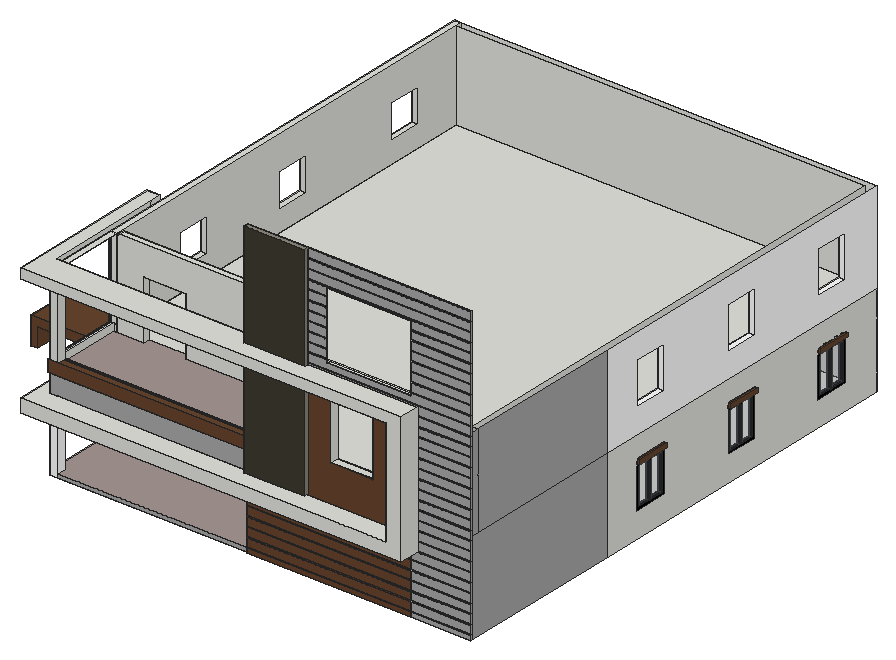
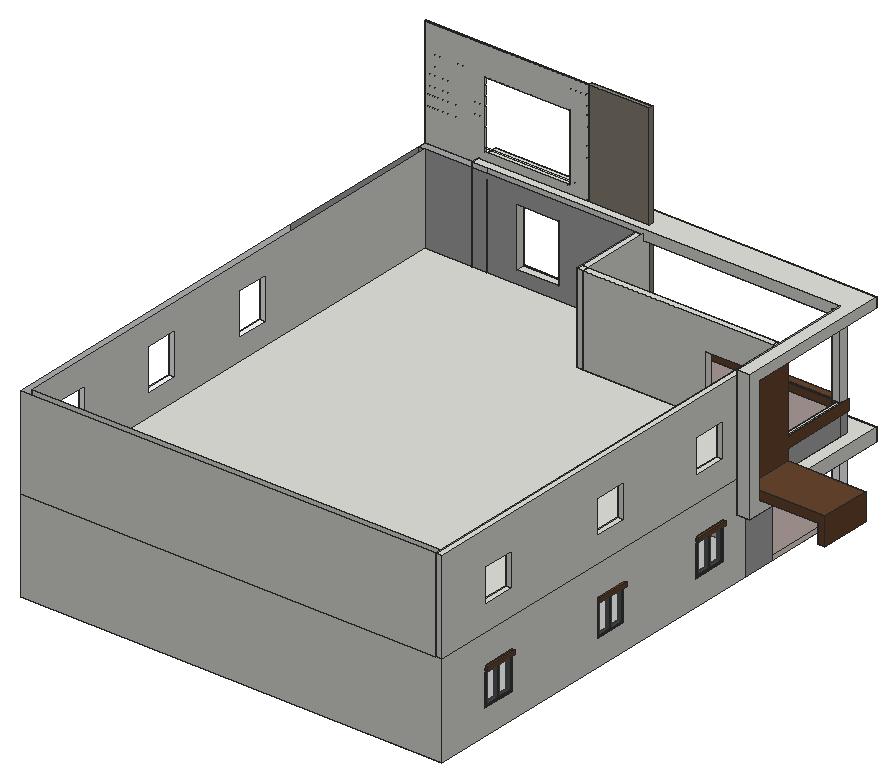
# SketchUp Ruby script. Lengths in inches.
U = 1.inch
M = Sketchup.active_model
def pt(a) = Geom::Point3d.new(a.map { |v| v * U })
def face(e, loops, mat)
  f = e.add_face(loops[0].map { |a| pt(a) })
  loops[1..].each { |l| e.add_face(l.map { |a| pt(a) }).erase! }
  f.material = f.back_material = mat if mat
  f
end
# faces: each face lists its corners as indices into pts; further lists are holes
def faces(e, pts, list, mat = nil) = list.each { |f| face(e, (f[0].is_a?(Array) ? f : [f]).map { |l| l.map { |i| pts[i] } }, mat) }
# xy, xz, yz: faces in a plane at the given z, y or x. An outline is a flat list of corners, or four numbers for a rectangle; further outlines are holes
def ring(l) = l.size == 4 ? [[l[0], l[1]], [l[2], l[1]], [l[2], l[3]], [l[0], l[3]]] : l.each_slice(2).to_a
def flat(e, list, mat, &to3) = list.each { |f| face(e, (f[0].is_a?(Array) ? f : [f]).map { |l| ring(l).map { |u, v| to3.(u, v) } }, mat) }
def xy(e, z, list, mat = nil) = flat(e, list, mat) { |x, y| [x, y, z] }
def xz(e, y, list, mat = nil) = flat(e, list, mat) { |x, z| [x, y, z] }
def yz(e, x, list, mat = nil) = flat(e, list, mat) { |y, z| [x, y, z] }
def lines(e, pts, list) = list.each { |a, b| e.add_line(pt(pts[a]), pt(pts[b])) }
# prism: a flat outline (further loops are holes) pulled along v
def prism(e, loops, v, mat = nil)
  f = face(e, loops, mat); d = Geom::Vector3d.new(v.map { |x| x * U })
  f.pushpull(f.normal.samedirection?(d) ? d.length : -d.length)
end
def box(e, o, s, mat = nil) = prism(e, [[o, [o[0] + s[0], o[1], o[2]], [o[0] + s[0], o[1] + s[1], o[2]], [o[0], o[1] + s[1], o[2]]]], [0, 0, s[2]], mat)
def at(x, y, z, deg = 0) = Geom::Transformation.translation(pt([x, y, z])) * Geom::Transformation.rotation(ORIGIN, Z_AXIS, deg.degrees)
def axes(o, x, y, z) = Geom::Transformation.new([*x, 0, *y, 0, *z, 0, *pt(o).to_a, 1])
def part(name) = M.definitions.add(name)
# library, detail: a bought-in or finely detailed component or shape, given as its bounding box
def library(name, o, s) = part(name).tap { |d| box(d.entities, o, s) }
def detail(e, o, s) = box(e.add_group.entities, o, s)
def put(e, d, t, mat = nil) = e.add_instance(d, t).tap { |i| i.material = mat if mat }
def group(e, t, mat = nil) = e.add_group.tap { |g| g.transformation = t; g.material = mat if mat }.entities
root = M.entities
M.materials.add("Glass_Basic_01").color = [161, 173, 186]
M.materials["Glass_Basic_01"].alpha = 0.25
M.materials.add("M00_Soft_Cloud").color = [255, 255, 255]
M.materials.add("M03_Pewter_Shine").color = [168, 168, 168]
M.materials.add("M07_Charcoal_Gleam").color = [58, 58, 58]
M.materials.add("M09_Shadow_Night").color = [0, 0, 0]
M.materials.add("Marble_01_1K").color = [230, 221, 211]
M.materials.add("Marble_06_1K").color = [165, 150, 147]
M.materials.add("Metal_06_1K").color = [238, 236, 231]
M.materials.add("Plaster_06_1K").color = [141, 135, 122]
M.materials.add("Tile_Exterior_07_1K").color = [112, 111, 107]
M.materials.add("Tile_Exterior_08_1K").color = [62, 60, 47]
M.materials.add("Wood_Veneer_15_1K").color = [103, 69, 45]
c1 = library("Group\#33",[0,0,0],[60,6,84])
c2 = part("Stair tread")
xy(c2.entities,3,[[0,0,10,60]],"Wood_Veneer_15_1K")
xy(c2.entities,6,[[0,0,10,60]],"Wood_Veneer_15_1K")
xz(c2.entities,0,[[0,3,10,6]],"Wood_Veneer_15_1K")
xz(c2.entities,60,[[0,3,10,6]])
yz(c2.entities,0,[[0,3,60,6]],"Wood_Veneer_15_1K")
yz(c2.entities,10,[[0,3,60,6]],"Wood_Veneer_15_1K")
c3 = part("Tread with baluster")
box(c3.entities,[0,0,3],[10,60,3])
g1 = group(c3.entities,at(3.7,1.6875,6))
prism(g1,[[[0.9375,0,0],[0.69,0.03,0],[0.47,0.125,0],[0.27,0.27,0],[0.125,0.47,0],[0.03,0.69,0],[0,0.9375,0],[0.03,1.18,0],[0.125,1.41,0],[0.27,1.6,0],[0.47,1.75,0],[0.69,1.84,0],[0.9375,1.875,0],[1.18,1.84,0],[1.41,1.75,0],[1.6,1.6,0],[1.75,1.41,0],[1.84,1.18,0],[1.875,0.9375,0],[1.84,0.69,0],[1.75,0.47,0],[1.6,0.27,0],[1.41,0.125,0],[1.18,0.03,0]]],[0,0,36.125],"Metal_06_1K")
c4 = part("Group\#49")
put(c4.entities,c2,at(70,0,87))
put(c4.entities,c2,at(60,0,93))
put(c4.entities,c2,at(30,0,111))
put(c4.entities,c2,at(90,0,75))
put(c4.entities,c2,at(10,0,123))
put(c4.entities,c2,at(20,0,117))
put(c4.entities,c2,at(50,0,99))
put(c4.entities,c2,at(40,0,105))
put(c4.entities,c2,at(100,0,69))
put(c4.entities,c2,at(80,0,81))
put(c4.entities,c3,at(100,60,57),"Wood_Veneer_15_1K")
put(c4.entities,c3,at(40,60,21),"Wood_Veneer_15_1K")
put(c4.entities,c3,at(60,60,33),"Wood_Veneer_15_1K")
put(c4.entities,c3,at(80,60,45),"Wood_Veneer_15_1K")
put(c4.entities,c3,at(90,60,51),"Wood_Veneer_15_1K")
put(c4.entities,c3,at(70,60,39),"Wood_Veneer_15_1K")
put(c4.entities,c3,at(10,60,3),"Wood_Veneer_15_1K")
put(c4.entities,c3,at(50,60,27),"Wood_Veneer_15_1K")
put(c4.entities,c3,at(30,60,15),"Wood_Veneer_15_1K")
put(c4.entities,c3,at(0,60,-3),"Wood_Veneer_15_1K")
put(c4.entities,c3,at(20,60,9),"Wood_Veneer_15_1K")
g2 = group(c4.entities,at(110,60,63),"Wood_Veneer_15_1K")
box(g2,[0,-60,0],[70,120,6])
c5 = part("Group\#23")
xy(c5.entities,0,[[-6,0,0,48]],"M07_Charcoal_Gleam")
xy(c5.entities,3,[[-6,3,0,23],[-6,25,0,45]],"M07_Charcoal_Gleam")
xy(c5.entities,45,[[-6,3,0,23],[-6,25,0,45]],"M07_Charcoal_Gleam")
xy(c5.entities,48,[[-6,0,0,48]],"M07_Charcoal_Gleam")
xz(c5.entities,0,[[-6,0,0,48]],"M07_Charcoal_Gleam")
xz(c5.entities,3,[[-6,3,0,45]],"M07_Charcoal_Gleam")
xz(c5.entities,23,[[-6,3,0,45]],"M07_Charcoal_Gleam")
xz(c5.entities,25,[[-6,3,0,45]],"M07_Charcoal_Gleam")
xz(c5.entities,45,[[-6,3,0,45]],"M07_Charcoal_Gleam")
xz(c5.entities,48,[[-6,0,0,48]],"M07_Charcoal_Gleam")
yz(c5.entities,-6,[[3,3,23,45],[25,3,45,45]],"Glass_Basic_01")
yz(c5.entities,-6,[[[0,0,48,48],[3,3,45,45]],[23,3,25,45]],"M07_Charcoal_Gleam")
yz(c5.entities,0,[[[0,0,48,48],[25,3,45,45],[3,3,23,45]]],"M07_Charcoal_Gleam")
c6 = part("Group\#21")
xy(c6.entities,0,[[0,0,6,48]],"M09_Shadow_Night")
xy(c6.entities,3,[[0,3,6,23],[0,25,6,45]],"M09_Shadow_Night")
xy(c6.entities,56.625,[[0,3,6,23],[0,25,6,45]],"M09_Shadow_Night")
xy(c6.entities,59.625,[[0,0,6,48]],"M09_Shadow_Night")
xz(c6.entities,0,[[0,0,6,59.625]],"M09_Shadow_Night")
xz(c6.entities,3,[[0,3,6,56.625]],"M09_Shadow_Night")
xz(c6.entities,23,[[0,3,6,56.625]],"M09_Shadow_Night")
xz(c6.entities,25,[[0,3,6,56.625]],"M09_Shadow_Night")
xz(c6.entities,45,[[0,3,6,56.625]],"M09_Shadow_Night")
xz(c6.entities,48,[[0,0,6,59.625]],"M09_Shadow_Night")
yz(c6.entities,0,[[[0,0,48,59.625],[25,3,45,56.625],[3,3,23,56.625]]],"M09_Shadow_Night")
yz(c6.entities,6,[[3,3,23,56.625],[25,3,45,56.625]],"Glass_Basic_01")
yz(c6.entities,6,[[[0,0,48,59.625],[3,3,45,56.625]],[23,3,25,56.625]],"M09_Shadow_Night")
c7 = part("Group\#22")
box(c7.entities,[-4,0,0],[4,48,6],"Wood_Veneer_15_1K")
g3 = group(root,at(8950.9375,4405.5625,18))
xy(g3,0,[[0,0,600,720]])
xy(g3,6,[[287.43,12,591,12,591,711,9,711,9,140.1,287.43,140.1]])
xy(g3,6,[[12,0,281.43,0,281.43,134.1,110.3125,134.1,110.3125,140.1,50.3125,140.1,50.3125,134.1,0,134.1,0,12,12,12]],"Marble_06_1K")
xy(g3,36,[[0,220.125,9,268.125],[591,294.5625,600,342.5625],[0,396.5,9,444.5],[591,456.0625,600,504.0625],[0,595.3125,9,643.3125],
  [591,616.5625,600,664.5625]])
xy(g3,84,[[0,220.125,9,268.125],[0,396.5,9,444.5],[0,595.3125,9,643.3125]])
xy(g3,90,[[50.3125,134.1,110.3125,140.1]])
xy(g3,96,[[591,294.5625,600,342.5625],[591,456.0625,600,504.0625],[591,616.5625,600,664.5625]])
xy(g3,104.53,[[12,0,281.43,12],[0,12,9,134.1],[9,12,281.43,134.1]])
xy(g3,131.625,[[0,0,12,0,12,6.5625,9,6.5625,9,12,0,12],[9,6.5625,12,12],[281.43,12,287.43,134.1],[9,134.1,287.43,140.1]])
xy(g3,132,[[12,0,600,0,600,720,0,720,0,12,9,12,9,711,591,711,591,12,12,12],[9,6.5625,12,12]])
xz(g3,0,[[0,0,12,95.53]],"M00_Soft_Cloud")
xz(g3,0,[[12,0,600,0,600,132,12,132,12,131.625,0,131.625,0,95.53,12,95.53,12,104.53,281.43,104.53,281.43,6,12,6]],"M03_Pewter_Shine")
xz(g3,6.5625,[[9,131.625,12,132]])
xz(g3,12,[[287.43,6,287.43,131.625,281.43,131.625,281.43,104.53,9,104.53,9,131.625,12,131.625,12,132,591,132,591,6],[0,131.625,9,132],[9,131.625,12,132]])
xz(g3,12,[[0,6,12,104.53]],"M00_Soft_Cloud")
xz(g3,134.1,[[0,6,50.3125,6,50.3125,90,110.3125,90,110.3125,6,281.43,6,281.43,104.53,0,104.53],[281.43,6,287.43,104.53],[9,104.53,281.43,131.625],[281.43,104.53,287.43,131.625]])
xz(g3,140.1,[[9,6,9,131.625,287.43,131.625,287.43,6,110.3125,6,110.3125,90,50.3125,90,50.3125,6]])
xz(g3,220.125,[[0,36,9,84]])
xz(g3,268.125,[[0,36,9,84]])
xz(g3,294.5625,[[591,36,600,96]])
xz(g3,342.5625,[[591,36,600,96]])
xz(g3,396.5,[[0,36,9,84]])
xz(g3,444.5,[[0,36,9,84]])
xz(g3,456.0625,[[591,36,600,96]])
xz(g3,504.0625,[[591,36,600,96]])
xz(g3,595.3125,[[0,36,9,84]])
xz(g3,616.5625,[[591,36,600,96]])
xz(g3,643.3125,[[0,36,9,84]])
xz(g3,664.5625,[[591,36,600,96]])
xz(g3,711,[[9,6,591,132]])
xz(g3,720,[[0,0,600,132]])
yz(g3,0,[[[179.8125,0,720,132],[220.125,36,268.125,84],[396.5,36,444.5,84],[595.3125,36,643.3125,84]]])
yz(g3,0,[[0,0,12,95.53]],"M00_Soft_Cloud")
yz(g3,0,[[134.1,0,134.1,104.53,12,104.53,12,132,179.8125,132,179.8125,0],[0,95.53,12,131.625]],"M03_Pewter_Shine")
yz(g3,0,[[12,0,134.1,6]],"Marble_01_1K")
yz(g3,9,[[[140.1,6,711,6,711,132,12,132,12,104.53,134.1,104.53,134.1,131.625,140.1,131.625],[220.125,36,268.125,84],[396.5,36,444.5,84],[595.3125,36,643.3125,84]],[6.5625,131.625,12,132]])
yz(g3,12,[[0,131.625,6.5625,132],[6.5625,131.625,12,132]])
yz(g3,12,[[0,6,12,104.53]],"M00_Soft_Cloud")
yz(g3,50.3125,[[134.1,6,140.1,90]])
yz(g3,110.3125,[[134.1,6,140.1,90]])
yz(g3,281.43,[[0,6,134.1,104.53],[12,104.53,134.1,131.625]])
yz(g3,287.43,[[12,6,134.1,131.625],[134.1,6,140.1,131.625]])
yz(g3,591,[[[12,6,711,132],[294.5625,36,342.5625,96],[456.0625,36,504.0625,96],[616.5625,36,664.5625,96]]])
yz(g3,600,[[[240,0,720,132],[294.5625,36,342.5625,96],[456.0625,36,504.0625,96],[616.5625,36,664.5625,96]]])
yz(g3,600,[[0,0,240,132]],"M03_Pewter_Shine")
g4 = group(root,at(9465.6,4405.5625,18))
xy(g4,0,[[0,-0.91,85.34,0]],"M03_Pewter_Shine")
xy(g4,6.0625,[[0,-0.91,85.34,-0.29]],"M09_Shadow_Night")
xy(g4,8.0625,[[0,-0.91,85.34,-0.29]],"M09_Shadow_Night")
xy(g4,19.37,[[0,-0.91,85.34,-0.29]],"M09_Shadow_Night")
xy(g4,21.37,[[0,-0.91,85.34,-0.29]],"M09_Shadow_Night")
xy(g4,32.68,[[0,-0.91,85.34,-0.29]],"M09_Shadow_Night")
xy(g4,34.68,[[0,-0.91,85.34,-0.29]],"M09_Shadow_Night")
xy(g4,45.98,[[0,-0.91,85.34,-0.29]],"M09_Shadow_Night")
xy(g4,47.98,[[0,-0.91,85.34,-0.29]],"M09_Shadow_Night")
xy(g4,59.29,[[0,-0.91,85.34,-0.29]],"M09_Shadow_Night")
xy(g4,61.29,[[0,-0.91,85.34,-0.29]],"M09_Shadow_Night")
xy(g4,72.59,[[0,-0.91,85.34,-0.29]],"M09_Shadow_Night")
xy(g4,74.59,[[0,-0.91,85.34,-0.29]],"M09_Shadow_Night")
xy(g4,85.9,[[0,-0.91,85.34,-0.29]],"M09_Shadow_Night")
xy(g4,87.9,[[0,-0.91,85.34,-0.29]],"M09_Shadow_Night")
xy(g4,99.21,[[0,-0.91,85.34,-0.29]],"M09_Shadow_Night")
xy(g4,101.21,[[0,-0.91,85.34,-0.29]],"M09_Shadow_Night")
xy(g4,112.51,[[0,-0.91,85.34,-0.29]],"M09_Shadow_Night")
xy(g4,114.51,[[0,-0.91,85.34,-0.29]],"M09_Shadow_Night")
xy(g4,125.82,[[0,-0.91,85.34,-0.29]],"M09_Shadow_Night")
xy(g4,127.82,[[0,-0.91,85.34,-0.29]],"M09_Shadow_Night")
xy(g4,139.125,[[0,-0.91,85.34,-0.29]],"M09_Shadow_Night")
xy(g4,141.125,[[0,-0.91,85.34,-0.29]],"M09_Shadow_Night")
xy(g4,152.43,[[0,-0.91,85.34,-0.29]],"M09_Shadow_Night")
xy(g4,154.43,[[0,-0.91,85.34,-0.29]],"M09_Shadow_Night")
xy(g4,165.74,[[0,-0.91,85.34,-0.29]],"M09_Shadow_Night")
xy(g4,167.74,[[0,-0.91,85.34,-0.29]],"M09_Shadow_Night")
xy(g4,179.04,[[0,-0.91,85.34,-0.29]],"M09_Shadow_Night")
xy(g4,181.04,[[0,-0.91,85.34,-0.29]],"M09_Shadow_Night")
xy(g4,192.35,[[0,-0.91,85.34,-0.29]],"M09_Shadow_Night")
xy(g4,194.35,[[0,-0.91,85.34,-0.29]],"M09_Shadow_Night")
xy(g4,205.66,[[0,-0.91,85.34,-0.29]],"M09_Shadow_Night")
xy(g4,207.66,[[0,-0.91,85.34,-0.29]],"M09_Shadow_Night")
xy(g4,218.96,[[0,-0.91,85.34,-0.29]],"M09_Shadow_Night")
xy(g4,220.96,[[0,-0.91,85.34,-0.29]],"M09_Shadow_Night")
xy(g4,232.27,[[0,-0.91,85.34,-0.29]],"M09_Shadow_Night")
xy(g4,234.27,[[0,-0.91,85.34,-0.29]],"M09_Shadow_Night")
xy(g4,245.57,[[0,-0.91,85.34,-0.29]],"M09_Shadow_Night")
xy(g4,247.57,[[0,-0.91,85.34,-0.29]],"M09_Shadow_Night")
xy(g4,258.88,[[0,-0.91,85.34,-0.29]],"M09_Shadow_Night")
xy(g4,260.88,[[0,-0.91,85.34,-0.29]],"M09_Shadow_Night")
xy(g4,263.25,[[-147.125,-0.91,0,0]])
xy(g4,272.1875,[[-147.125,-0.91,85.34,-0.29]],"M09_Shadow_Night")
xy(g4,274.1875,[[-147.125,-0.91,85.34,-0.29]],"M09_Shadow_Night")
xy(g4,281.625,[[-120.5,-0.91,0,0]])
xy(g4,285.49,[[-147.125,-0.91,-120.5,-0.29],[0,-0.91,85.34,-0.29]],"M09_Shadow_Night")
xy(g4,287.49,[[-147.125,-0.91,-120.5,-0.29],[0,-0.91,85.34,-0.29]],"M09_Shadow_Night")
xy(g4,298.8,[[-147.125,-0.91,-120.5,-0.29],[0,-0.91,85.34,-0.29]],"M09_Shadow_Night")
xy(g4,300.8,[[-147.125,-0.91,-120.5,-0.29],[0,-0.91,85.34,-0.29]],"M09_Shadow_Night")
xy(g4,312.11,[[-147.125,-0.91,-120.5,-0.29],[0,-0.91,85.34,-0.29]],"M09_Shadow_Night")
xy(g4,314.11,[[-147.125,-0.91,-120.5,-0.29],[0,-0.91,85.34,-0.29]],"M09_Shadow_Night")
xy(g4,325.41,[[-147.125,-0.91,-120.5,-0.29],[0,-0.91,85.34,-0.29]],"M09_Shadow_Night")
xy(g4,327.41,[[-147.125,-0.91,-120.5,-0.29],[0,-0.91,85.34,-0.29]],"M09_Shadow_Night")
xy(g4,338.72,[[-147.125,-0.91,-120.5,-0.29],[0,-0.91,85.34,-0.29]],"M09_Shadow_Night")
xy(g4,340.72,[[-147.125,-0.91,-120.5,-0.29],[0,-0.91,85.34,-0.29]],"M09_Shadow_Night")
xy(g4,352.02,[[-147.125,-0.91,-120.5,-0.29],[0,-0.91,85.34,-0.29]],"M09_Shadow_Night")
xy(g4,354.02,[[-147.125,-0.91,-120.5,-0.29],[0,-0.91,85.34,-0.29]],"M09_Shadow_Night")
xy(g4,365.33,[[-147.125,-0.91,-120.5,-0.29],[0,-0.91,85.34,-0.29]],"M09_Shadow_Night")
xy(g4,367.33,[[-147.125,-0.91,-120.5,-0.29],[0,-0.91,85.34,-0.29]],"M09_Shadow_Night")
xy(g4,377.625,[[-120.5,-0.91,0,0]])
xy(g4,378.64,[[-147.125,-0.91,85.34,-0.29]],"M09_Shadow_Night")
xy(g4,380.64,[[-147.125,-0.91,85.34,-0.29]],"M09_Shadow_Night")
xy(g4,391.94,[[-147.125,-0.91,85.34,-0.29]],"M09_Shadow_Night")
xy(g4,393.94,[[-147.125,-0.91,85.34,-0.29]],"M09_Shadow_Night")
xy(g4,405.25,[[-147.125,-0.91,85.34,-0.29]],"M09_Shadow_Night")
xy(g4,407.25,[[-147.125,-0.91,85.34,-0.29]],"M09_Shadow_Night")
xy(g4,419.25,[[-147.125,-0.91,85.34,0]])
xz(g4,-0.91,[[0,0,85.34,6.0625],[0,8.0625,85.34,19.37],[0,21.37,85.34,32.68],[0,34.68,85.34,45.98],[0,47.98,85.34,59.29],
  [0,61.29,85.34,72.59],[0,74.59,85.34,85.9],[0,87.9,85.34,99.21],[0,101.21,85.34,112.51],[0,114.51,85.34,125.82],
  [0,127.82,85.34,139.125],[0,141.125,85.34,152.43],[0,154.43,85.34,165.74],[0,167.74,85.34,179.04],[0,181.04,85.34,192.35],
  [0,194.35,85.34,205.66],[0,207.66,85.34,218.96],[0,220.96,85.34,232.27],[0,234.27,85.34,245.57],[0,247.57,85.34,258.88],
  [0,260.88,85.34,260.88,85.34,272.1875,-147.125,272.1875,-147.125,263.25,0,263.25],[-147.125,274.1875,85.34,274.1875,85.34,285.49,0,285.49,0,281.625,-120.5,281.625,-120.5,285.49,-147.125,285.49],[-147.125,287.49,-120.5,298.8],[0,287.49,85.34,298.8],[-147.125,300.8,-120.5,312.11],
  [0,300.8,85.34,312.11],[-147.125,314.11,-120.5,325.41],[0,314.11,85.34,325.41],[-147.125,327.41,-120.5,338.72],[0,327.41,85.34,338.72],
  [-147.125,340.72,-120.5,352.02],[0,340.72,85.34,352.02],[-147.125,354.02,-120.5,365.33],[0,354.02,85.34,365.33],[-147.125,367.33,-120.5,367.33,-120.5,377.625,0,377.625,0,367.33,85.34,367.33,85.34,378.64,-147.125,378.64],
  [-147.125,380.64,85.34,391.94],[-147.125,393.94,85.34,405.25],[-147.125,407.25,85.34,419.25]],"M03_Pewter_Shine")
xz(g4,-0.29,[[0,6.0625,85.34,8.0625],[0,19.37,85.34,21.37],[0,32.68,85.34,34.68],[0,45.98,85.34,47.98],[0,59.29,85.34,61.29],
  [0,72.59,85.34,74.59],[0,85.9,85.34,87.9],[0,99.21,85.34,101.21],[0,112.51,85.34,114.51],[0,125.82,85.34,127.82],
  [0,139.125,85.34,141.125],[0,152.43,85.34,154.43],[0,165.74,85.34,167.74],[0,179.04,85.34,181.04],[0,192.35,85.34,194.35],
  [0,205.66,85.34,207.66],[0,218.96,85.34,220.96],[0,232.27,85.34,234.27],[0,245.57,85.34,247.57],[0,258.88,85.34,260.88],
  [-147.125,272.1875,85.34,274.1875],[-147.125,285.49,-120.5,287.49],[0,285.49,85.34,287.49],[-147.125,298.8,-120.5,300.8],[0,298.8,85.34,300.8],
  [-147.125,312.11,-120.5,314.11],[0,312.11,85.34,314.11],[-147.125,325.41,-120.5,327.41],[0,325.41,85.34,327.41],[-147.125,338.72,-120.5,340.72],
  [0,338.72,85.34,340.72],[-147.125,352.02,-120.5,354.02],[0,352.02,85.34,354.02],[-147.125,365.33,-120.5,367.33],[0,365.33,85.34,367.33],
  [-147.125,378.64,85.34,380.64],[-147.125,391.94,85.34,393.94],[-147.125,405.25,85.34,407.25]],"M09_Shadow_Night")
xz(g4,0,[[[0,0,0,263.25,-147.125,263.25,-147.125,419.25,85.34,419.25,85.34,0],[-120.5,281.625,0,377.625]]])
yz(g4,-147.125,[[-0.91,263.25,-0.91,272.1875,-0.29,272.1875,-0.29,274.1875,-0.91,274.1875,-0.91,285.49,-0.29,285.49,-0.29,287.49,-0.91,287.49,-0.91,298.8,-0.29,298.8,-0.29,300.8,-0.91,300.8,-0.91,312.11,-0.29,312.11,-0.29,314.11,-0.91,314.11,-0.91,325.41,-0.29,325.41,-0.29,327.41,-0.91,327.41,-0.91,338.72,-0.29,338.72,-0.29,340.72,-0.91,340.72,-0.91,352.02,-0.29,352.02,-0.29,354.02,-0.91,354.02,-0.91,365.33,-0.29,365.33,-0.29,367.33,-0.91,367.33,-0.91,377.625,0,377.625,0,263.25],[-0.91,377.625,-0.91,378.64,-0.29,378.64,-0.29,380.64,-0.91,380.64,-0.91,391.94,-0.29,391.94,-0.29,393.94,-0.91,393.94,-0.91,405.25,-0.29,405.25,-0.29,407.25,-0.91,407.25,-0.91,419.25,0,419.25,0,377.625]])
yz(g4,-120.5,[[-0.91,281.625,0,281.625,0,377.625,-0.91,377.625,-0.91,367.33,-0.29,367.33,-0.29,365.33,-0.91,365.33,-0.91,354.02,-0.29,354.02,-0.29,352.02,-0.91,352.02,-0.91,340.72,-0.29,340.72,-0.29,338.72,-0.91,338.72,-0.91,327.41,-0.29,327.41,-0.29,325.41,-0.91,325.41,-0.91,314.11,-0.29,314.11,-0.29,312.11,-0.91,312.11,-0.91,300.8,-0.29,300.8,-0.29,298.8,-0.91,298.8,-0.91,287.49,-0.29,287.49,-0.29,285.49,-0.91,285.49]])
yz(g4,0,[[-0.91,0,-0.91,6.0625,-0.29,6.0625,-0.29,8.0625,-0.91,8.0625,-0.91,19.37,-0.29,19.37,-0.29,21.37,-0.91,21.37,-0.91,32.68,-0.29,32.68,-0.29,34.68,-0.91,34.68,-0.91,45.98,-0.29,45.98,-0.29,47.98,-0.91,47.98,-0.91,59.29,-0.29,59.29,-0.29,61.29,-0.91,61.29,-0.91,72.59,-0.29,72.59,-0.29,74.59,-0.91,74.59,-0.91,85.9,-0.29,85.9,-0.29,87.9,-0.91,87.9,-0.91,99.21,-0.29,99.21,-0.29,101.21,-0.91,101.21,-0.91,112.51,-0.29,112.51,-0.29,114.51,-0.91,114.51,-0.91,125.82,-0.29,125.82,-0.29,127.82,-0.91,127.82,-0.91,139.125,-0.29,139.125,-0.29,141.125,-0.91,141.125,-0.91,152.43,-0.29,152.43,-0.29,154.43,-0.91,154.43,-0.91,165.74,-0.29,165.74,-0.29,167.74,-0.91,167.74,-0.91,179.04,-0.29,179.04,-0.29,181.04,-0.91,181.04,-0.91,192.35,-0.29,192.35,-0.29,194.35,-0.91,194.35,-0.91,205.66,-0.29,205.66,-0.29,207.66,-0.91,207.66,-0.91,218.96,-0.29,218.96,-0.29,220.96,-0.91,220.96,-0.91,232.27,-0.29,232.27,-0.29,234.27,-0.91,234.27,-0.91,245.57,-0.29,245.57,-0.29,247.57,-0.91,247.57,-0.91,258.88,-0.29,258.88,-0.29,260.88,-0.91,260.88,-0.91,263.25,0,263.25,0,0],[-0.91,281.625,-0.91,285.49,-0.29,285.49,-0.29,287.49,-0.91,287.49,-0.91,298.8,-0.29,298.8,-0.29,300.8,-0.91,300.8,-0.91,312.11,-0.29,312.11,-0.29,314.11,-0.91,314.11,-0.91,325.41,-0.29,325.41,-0.29,327.41,-0.91,327.41,-0.91,338.72,-0.29,338.72,-0.29,340.72,-0.91,340.72,-0.91,352.02,-0.29,352.02,-0.29,354.02,-0.91,354.02,-0.91,365.33,-0.29,365.33,-0.29,367.33,-0.91,367.33,-0.91,377.625,0,377.625,0,281.625]])
yz(g4,85.34,[[-0.91,0,0,0,0,419.25,-0.91,419.25,-0.91,407.25,-0.29,407.25,-0.29,405.25,-0.91,405.25,-0.91,393.94,-0.29,393.94,-0.29,391.94,-0.91,391.94,-0.91,380.64,-0.29,380.64,-0.29,378.64,-0.91,378.64,-0.91,367.33,-0.29,367.33,-0.29,365.33,-0.91,365.33,-0.91,354.02,-0.29,354.02,-0.29,352.02,-0.91,352.02,-0.91,340.72,-0.29,340.72,-0.29,338.72,-0.91,338.72,-0.91,327.41,-0.29,327.41,-0.29,325.41,-0.91,325.41,-0.91,314.11,-0.29,314.11,-0.29,312.11,-0.91,312.11,-0.91,300.8,-0.29,300.8,-0.29,298.8,-0.91,298.8,-0.91,287.49,-0.29,287.49,-0.29,285.49,-0.91,285.49,-0.91,274.1875,-0.29,274.1875,-0.29,272.1875,-0.91,272.1875,-0.91,260.88,-0.29,260.88,-0.29,258.88,-0.91,258.88,-0.91,247.57,-0.29,247.57,-0.29,245.57,-0.91,245.57,-0.91,234.27,-0.29,234.27,-0.29,232.27,-0.91,232.27,-0.91,220.96,-0.29,220.96,-0.29,218.96,-0.91,218.96,-0.91,207.66,-0.29,207.66,-0.29,205.66,-0.91,205.66,-0.91,194.35,-0.29,194.35,-0.29,192.35,-0.91,192.35,-0.91,181.04,-0.29,181.04,-0.29,179.04,-0.91,179.04,-0.91,167.74,-0.29,167.74,-0.29,165.74,-0.91,165.74,-0.91,154.43,-0.29,154.43,-0.29,152.43,-0.91,152.43,-0.91,141.125,-0.29,141.125,-0.29,139.125,-0.91,139.125,-0.91,127.82,-0.29,127.82,-0.29,125.82,-0.91,125.82,-0.91,114.51,-0.29,114.51,-0.29,112.51,-0.91,112.51,-0.91,101.21,-0.29,101.21,-0.29,99.21,-0.91,99.21,-0.91,87.9,-0.29,87.9,-0.29,85.9,-0.91,85.9,-0.91,74.59,-0.29,74.59,-0.29,72.59,-0.91,72.59,-0.91,61.29,-0.29,61.29,-0.29,59.29,-0.91,59.29,-0.91,47.98,-0.29,47.98,-0.29,45.98,-0.91,45.98,-0.91,34.68,-0.29,34.68,-0.29,32.68,-0.91,32.68,-0.91,21.37,-0.29,21.37,-0.29,19.37,-0.91,19.37,-0.91,8.0625,-0.29,8.0625,-0.29,6.0625,-0.91,6.0625]],"M03_Pewter_Shine")
p = [[0,-0.91,285.49],[-120.5,-0.91,285.49],[0,-0.91,287.49],[-120.5,-0.91,287.49],[0,-0.91,258.88],[-147.125,-0.91,258.88],
  [0,-0.91,260.88],[-147.125,-0.91,260.88],[0,-0.91,99.21],[-147.125,-0.91,99.21],[0,-0.91,101.21],[-147.125,-0.91,101.21]]
lines(g4,p,[[0,1],[2,3],[4,5],[6,7],[8,9],[10,11]])
g5 = group(root,at(9232.37,4405.5625,18))
prism(g5,[[[0,0,95.53],[0,0,0],[0,-0.91,0],[0,-0.91,6.12],[0,-0.29,6.12],[0,-0.29,8.0625],[0,-0.91,8.0625],[0,-0.91,19.37],[0,-0.29,19.37],[0,-0.29,21.37],[0,-0.91,21.37],[0,-0.91,32.68],[0,-0.29,32.68],[0,-0.29,34.68],[0,-0.91,34.68],[0,-0.91,45.98],[0,-0.29,45.98],[0,-0.29,47.98],[0,-0.91,47.98],[0,-0.91,59.29],[0,-0.29,59.29],[0,-0.29,61.29],[0,-0.91,61.29],[0,-0.91,72.59],[0,-0.29,72.59],[0,-0.29,74.59],[0,-0.91,74.59],[0,-0.91,85.9],[0,-0.29,85.9],[0,-0.29,87.9],[0,-0.91,87.9],[0,-0.91,95.53]]],[233.23,0,0],"Wood_Veneer_15_1K")
put(root,c1,at(9001.25,4539.66,24))
put(root,c4,at(9361.9375,4417.5625,24))
g6 = group(root,at(8956.9375,4625.6875,54))
xy(g6,0,[[-6,0,0,48]],"M07_Charcoal_Gleam")
xy(g6,3,[[-6,3,0,23],[-6,25,0,45]],"M07_Charcoal_Gleam")
xy(g6,45,[[-6,3,0,23],[-6,25,0,45]],"M07_Charcoal_Gleam")
xy(g6,48,[[-6,0,0,48]],"M07_Charcoal_Gleam")
xz(g6,0,[[-6,0,0,48]],"M07_Charcoal_Gleam")
xz(g6,3,[[-6,3,0,45]],"M07_Charcoal_Gleam")
xz(g6,23,[[-6,3,0,45]],"M07_Charcoal_Gleam")
xz(g6,25,[[-6,3,0,45]],"M07_Charcoal_Gleam")
xz(g6,45,[[-6,3,0,45]],"M07_Charcoal_Gleam")
xz(g6,48,[[-6,0,0,48]],"M07_Charcoal_Gleam")
yz(g6,-6,[[3,3,23,45],[25,3,45,45]],"Glass_Basic_01")
yz(g6,-6,[[[0,0,48,48],[3,3,45,45]],[23,3,25,45]],"M07_Charcoal_Gleam")
yz(g6,0,[[[0,0,48,48],[25,3,45,45],[3,3,23,45]]],"M07_Charcoal_Gleam")
put(root,c5,at(8956.9375,4802.0625,54))
put(root,c5,at(8956.9375,5000.875,54))
put(root,c6,at(9544.9375,4700.125,54))
put(root,c6,at(9544.9375,4861.625,54))
put(root,c6,at(9544.9375,5022.125,54))
g7 = group(root,at(8950.9375,4405.5625,149.625))
xy(g7,0,[[15.25,-2,281.43,12],[0,0,0,108,9,108,9,720,600,720,600,12,12,12,12,0],[0,108,9,720]])
xy(g7,0,[[281.43,0,600,12]],"M03_Pewter_Shine")
xy(g7,6,[[290.43,12,591,12,591,711,9,711,9,117,290.43,117],[281.43,12,290.43,108],[9,108,47.08,117],[107.08,108,281.43,117],[281.43,108,290.43,117]])
xy(g7,6,[[4.6875,12,281.43,12,281.43,108,107.08,108,107.08,117,47.08,117,47.08,108,4.6875,108]],"Marble_06_1K")
xy(g7,16,[[281.43,0,290.43,12],[0,12,4.6875,108]])
xy(g7,24.375,[[400.16,0,460.16,12]])
xy(g7,36,[[0,220.125,9,268.125],[0,396.5,9,444.5],[0,595.3125,9,643.3125]])
xy(g7,36.375,[[591,294.5625,600,342.5625],[591,456.0625,600,504.0625],[591,616.5625,600,664.5625]],"M00_Soft_Cloud")
xy(g7,84,[[0,220.125,9,268.125],[0,396.5,9,444.5],[0,595.3125,9,643.3125]])
xy(g7,90,[[47.08,108,107.08,117]])
xy(g7,96,[[591,294.5625,600,342.5625],[591,456.0625,600,504.0625],[591,616.5625,600,664.5625]],"M00_Soft_Cloud")
xy(g7,108,[[400.16,0,460.16,12]])
xy(g7,131.625,[[0,0,12,12],[0,12,9,108],[9,108,12,117]])
xy(g7,132,[[281.43,0,290.43,12],[0,12,9,720],[281.43,12,290.43,108],[12,108,281.43,117],[281.43,108,290.43,117]])
xy(g7,132,[[290.43,0,600,12]],"M03_Pewter_Shine")
xz(g7,0,[[0,0,12,131.625],[281.43,16,290.43,132]])
xz(g7,0,[[[281.43,0,600,0,600,132,290.43,132,290.43,16,281.43,16],[400.16,24.375,460.16,108]]],"M03_Pewter_Shine")
xz(g7,12,[[12,0,15.25,6],[15.25,0,281.43,6],[4.6875,6,4.6875,16,0,16,0,131.625,12,131.625,12,6],[281.43,6,290.43,16],[0,131.625,9,132],
  [9,131.625,12,132]])
xz(g7,12,[[[290.43,6,591,132],[400.16,24.375,460.16,108]]],"M03_Pewter_Shine")
xz(g7,108,[[0,0,9,0,9,6,4.6875,6,4.6875,16,0,16],[4.6875,6,9,16],[9,6,47.08,6,47.08,90,107.08,90,107.08,6,281.43,6,281.43,132,12,132,12,131.625,9,131.625],[281.43,6,290.43,132],[0,16,9,131.625]])
xz(g7,117,[[9,6,9,131.625,12,131.625,12,132,281.43,132,281.43,6,107.08,6,107.08,90,47.08,90,47.08,6],[281.43,6,290.43,132]])
xz(g7,220.125,[[0,36,9,84]])
xz(g7,268.125,[[0,36,9,84]])
xz(g7,294.5625,[[591,36.375,600,96]],"M00_Soft_Cloud")
xz(g7,342.5625,[[591,36.375,600,96]],"M00_Soft_Cloud")
xz(g7,396.5,[[0,36,9,84]])
xz(g7,444.5,[[0,36,9,84]])
xz(g7,456.0625,[[591,36.375,600,96]],"M00_Soft_Cloud")
xz(g7,504.0625,[[591,36.375,600,96]],"M00_Soft_Cloud")
xz(g7,595.3125,[[0,36,9,84]])
xz(g7,616.5625,[[591,36.375,600,96]],"M00_Soft_Cloud")
xz(g7,643.3125,[[0,36,9,84]])
xz(g7,664.5625,[[591,36.375,600,96]],"M00_Soft_Cloud")
xz(g7,711,[[9,6,591,132]])
xz(g7,720,[[0,0,9,132],[9,0,600,132]])
yz(g7,0,[[0,0,12,131.625],[12,0,108,16],[[108,0,108,131.625,12,131.625,12,132,720,132,720,0],[220.125,36,268.125,84],[396.5,36,444.5,84],[595.3125,36,643.3125,84]]])
yz(g7,4.6875,[[12,6,108,16]])
yz(g7,9,[[108,0,720,0,720,132,711,132,711,6,108,6],[[117,6,711,6,711,132,12,132,12,131.625,117,131.625],[220.125,36,268.125,84],[396.5,36,444.5,84],[595.3125,36,643.3125,84]],[108,6,117,16],[108,16,117,131.625]])
yz(g7,12,[[0,0,12,131.625],[108,131.625,117,132]])
yz(g7,47.08,[[108,6,117,90]])
yz(g7,107.08,[[108,6,117,90]])
yz(g7,281.43,[[-2,0,0,16],[0,0,12,16],[12,6,12,16,0,16,0,132,108,132,108,6],[108,6,117,132]])
yz(g7,290.43,[[12,6,108,132],[108,6,117,132]])
yz(g7,290.43,[[0,16,12,132]],"M03_Pewter_Shine")
yz(g7,400.16,[[0,24.375,12,108]])
yz(g7,460.16,[[0,24.375,12,108]])
yz(g7,591,[[[12,6,711,132],[294.5625,36.375,342.5625,96],[456.0625,36.375,504.0625,96],[616.5625,36.375,664.5625,96]]])
yz(g7,600,[[[240,0,720,132],[294.5625,36.375,342.5625,96],[456.0625,36.375,504.0625,96],[616.5625,36.375,664.5625,96]]],"M00_Soft_Cloud")
yz(g7,600,[[0,0,12,132],[12,0,240,132]],"M03_Pewter_Shine")
g8 = group(g7,at(15.25,-2,0),"Wood_Veneer_15_1K")
xy(g8,-53.625,[[-128.3125,110,-118.3125,181.8125]])
xy(g8,-27.1,[[-118.3125,110,-15.25,181.8125]])
xy(g8,-15.125,[[-128.3125,110,-17.25,181.8125],[-17.25,110,-15.25,181.8125]])
xy(g8,0,[[-17.25,0,-17.25,110,-15.25,110,-15.25,14,0,14,0,0]])
xy(g8,6,[[-15.25,11,266.18,14]])
xy(g8,16,[[-17.25,0,266.18,0,266.18,11,-15.25,11,-15.25,110,-17.25,110],[-15.25,11,266.18,14]])
xy(g8,124.625,[[-17.25,110,-15.25,181.8125]])
xz(g8,0,[[-17.25,0,266.18,16]])
xz(g8,11,[[-15.25,6,266.18,16]])
xz(g8,14,[[-15.25,6,266.18,16]])
xz(g8,110,[[-128.3125,-53.625,-118.3125,-53.625,-118.3125,-27.1,-15.25,-27.1,-15.25,-15.125,-128.3125,-15.125],[-17.25,-15.125,-15.25,0],[-17.25,16,-15.25,124.625]])
xz(g8,181.8125,[[-128.3125,-53.625,-128.3125,-15.125,-15.25,-15.125,-15.25,-27.1,-118.3125,-27.1,-118.3125,-53.625],[-17.25,-15.125,-15.25,124.625]])
yz(g8,-128.3125,[[110,-53.625,181.8125,-15.125]])
yz(g8,-118.3125,[[110,-53.625,181.8125,-27.1]])
yz(g8,-17.25,[[110,-15.125,110,0,0,0,0,16,110,16,110,124.625,181.8125,124.625,181.8125,-15.125]])
yz(g8,-15.25,[[110,-27.1,181.8125,-15.125],[110,-15.125,181.8125,-15.125,181.8125,6,14,6,14,0,110,0],[11,6,14,16],[14,6,181.8125,6,181.8125,124.625,110,124.625,110,16,14,16]])
yz(g8,266.18,[[11,6,14,16]])
put(root,c7,at(8950.9375,4625.6875,102))
put(root,c7,at(8950.9375,4802.0625,102))
put(root,c7,at(8950.9375,5000.875,102))
g9 = group(root,at(9111.18,4405.5625,281.25))
xy(g9,-176.97,[[-178.3125,-30,-178.3125,195.8125,-160.3125,195.8125,-160.3125,179.8125,-160.24,179.8125,-160.24,11.6875,363.67,11.6875,363.67,-30]])
xy(g9,-158.72,[[-178.3125,-30,342.42,-30,342.42,11.6875,-160.24,11.6875,-160.24,179.8125,-178.3125,179.8125]])
xy(g9,-7,[[-178.3125,-30,-178.3125,179.8125,-160.3125,179.8125,-160.3125,11.6875,342.42,11.6875,342.42,-30]])
xy(g9,7.4375,[[-178.3125,-30,363.67,-30,363.67,11.6875,-160.3125,11.6875,-160.3125,195.8125,-178.3125,195.8125]])
xz(g9,-30,[[-178.3125,-176.97,363.67,-176.97,363.67,7.4375,-178.3125,7.4375,-178.3125,-7,342.42,-7,342.42,-158.72,-178.3125,-158.72]])
xz(g9,11.6875,[[-160.24,-176.97,363.67,-158.72],[342.42,-158.72,363.67,7.4375],[-160.3125,-7,342.42,7.4375]])
xz(g9,179.8125,[[-160.3125,-176.97,-160.24,-158.72],[-178.3125,-158.72,-160.3125,-7]])
xz(g9,195.8125,[[-178.3125,-176.97,-160.3125,7.4375]])
yz(g9,-178.3125,[[-30,-176.97,-30,-158.72,179.8125,-158.72,179.8125,-7,-30,-7,-30,7.4375,195.8125,7.4375,195.8125,-176.97]])
yz(g9,-160.3125,[[179.8125,-176.97,195.8125,7.4375],[11.6875,-7,179.8125,7.4375]])
yz(g9,-160.24,[[11.6875,-176.97,179.8125,-158.72]])
yz(g9,342.42,[[-30,-158.72,11.6875,-7]])
yz(g9,363.67,[[-30,-176.97,11.6875,7.4375]])
put(root,c7,at(9554.9375,5022.125,114))
put(root,c7,at(9554.9375,4861.625,114))
put(root,c7,at(9554.9375,4700.125,114))
g10 = group(root,at(9232.37,4405.5625,149.625),"Tile_Exterior_07_1K")
xy(g10,-27.1,[[0,-6,86.1,0]],"Plaster_06_1K")
xy(g10,287.625,[[0,-6,86.1,0]],"Plaster_06_1K")
xz(g10,-6,[[0,-27.1,86.1,287.625]],"Tile_Exterior_08_1K")
xz(g10,0,[[0,-27.1,86.1,287.625]],"Plaster_06_1K")
yz(g10,0,[[-6,-27.1,0,287.625]],"Plaster_06_1K")
yz(g10,86.1,[[-6,-27.1,0,287.625]],"Plaster_06_1K")
g11 = group(root,at(9318.47,4405.5625,122.53))
xy(g11,0,[[0,-0.91,135.125,0]])
xy(g11,51.47,[[32.625,-0.91,92.625,0]])
xy(g11,135.1,[[32.625,-0.91,92.625,0]])
xy(g11,151.72,[[0,-0.91,135.125,0]])
xz(g11,-0.91,[[[0,0,135.125,151.72],[32.625,51.47,92.625,135.1]]],"Wood_Veneer_15_1K")
xz(g11,0,[[[0,0,135.125,151.72],[32.625,51.47,92.625,135.1]]])
yz(g11,0,[[-0.91,0,0,151.72]])
yz(g11,32.625,[[-0.91,51.47,0,135.1]])
yz(g11,92.625,[[-0.91,51.47,0,135.1]])
yz(g11,135.125,[[-0.91,0,0,151.72]])
